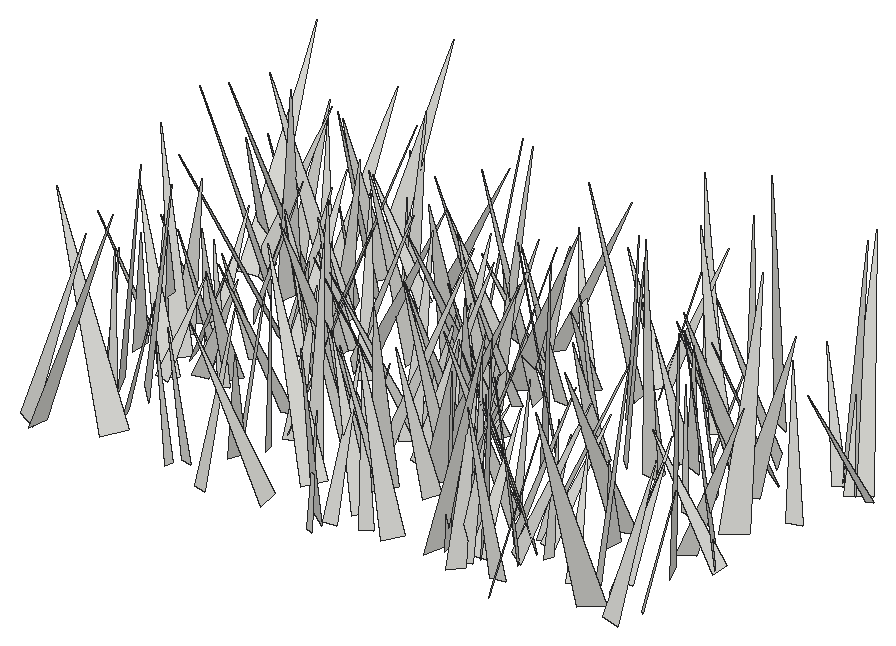
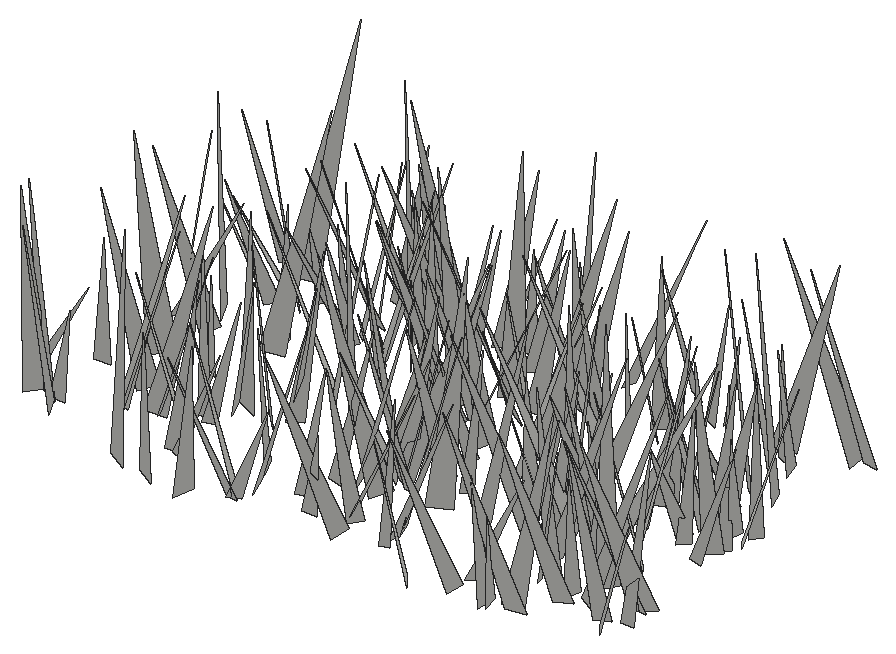
# SketchUp Ruby script. Lengths in inches.
U = 1.inch
M = Sketchup.active_model
def pt(a) = Geom::Point3d.new(a.map { |v| v * U })
def face(e, loops, mat)
  f = e.add_face(loops[0].map { |a| pt(a) })
  loops[1..].each { |l| e.add_face(l.map { |a| pt(a) }).erase! }
  f.material = f.back_material = mat if mat
  f
end
# faces: each face lists its corners as indices into pts; further lists are holes
def faces(e, pts, list, mat = nil) = list.each { |f| face(e, (f[0].is_a?(Array) ? f : [f]).map { |l| l.map { |i| pts[i] } }, mat) }
# xy, xz, yz: faces in a plane at the given z, y or x. An outline is a flat list of corners, or four numbers for a rectangle; further outlines are holes
def ring(l) = l.size == 4 ? [[l[0], l[1]], [l[2], l[1]], [l[2], l[3]], [l[0], l[3]]] : l.each_slice(2).to_a
def flat(e, list, mat, &to3) = list.each { |f| face(e, (f[0].is_a?(Array) ? f : [f]).map { |l| ring(l).map { |u, v| to3.(u, v) } }, mat) }
def xy(e, z, list, mat = nil) = flat(e, list, mat) { |x, y| [x, y, z] }
def xz(e, y, list, mat = nil) = flat(e, list, mat) { |x, z| [x, y, z] }
def yz(e, x, list, mat = nil) = flat(e, list, mat) { |y, z| [x, y, z] }
def lines(e, pts, list) = list.each { |a, b| e.add_line(pt(pts[a]), pt(pts[b])) }
# prism: a flat outline (further loops are holes) pulled along v
def prism(e, loops, v, mat = nil)
  f = face(e, loops, mat); d = Geom::Vector3d.new(v.map { |x| x * U })
  f.pushpull(f.normal.samedirection?(d) ? d.length : -d.length)
end
def box(e, o, s, mat = nil) = prism(e, [[o, [o[0] + s[0], o[1], o[2]], [o[0] + s[0], o[1] + s[1], o[2]], [o[0], o[1] + s[1], o[2]]]], [0, 0, s[2]], mat)
def at(x, y, z, deg = 0) = Geom::Transformation.translation(pt([x, y, z])) * Geom::Transformation.rotation(ORIGIN, Z_AXIS, deg.degrees)
def axes(o, x, y, z) = Geom::Transformation.new([*x, 0, *y, 0, *z, 0, *pt(o).to_a, 1])
def part(name) = M.definitions.add(name)
# library, detail: a bought-in or finely detailed component or shape, given as its bounding box
def library(name, o, s) = part(name).tap { |d| box(d.entities, o, s) }
def detail(e, o, s) = box(e.add_group.entities, o, s)
def put(e, d, t, mat = nil) = e.add_instance(d, t).tap { |i| i.material = mat if mat }
def group(e, t, mat = nil) = e.add_group.tap { |g| g.transformation = t; g.material = mat if mat }.entities
root = M.entities
c1 = part("fur_instance\#9")
p = [[0.8125,0,1.79],[0.67,-0.02,1.48],[0,-0.11,0],[0,0.11,0]]
faces(c1.entities,p,[[0,1,2,3]])
put(root,c1,axes([476.15,435.58,-21.66],[-2.86307,-5.78602,1.82095],[-5.78172,3.21211,1.11581],[1.83453,1.09334,6.35847]))
put(root,c1,axes([472.6,435.43,-21.66],[-6.27523,-0.24227,0.55286],[-0.1392,6.19931,1.13667],[0.58735,-1.11924,6.17618]))
put(root,c1,axes([495.21,437.4,-21.66],[3.52334,-7.25518,1.10129],[-7.15699,-3.66725,-1.26216],[-1.62106,0.42196,7.96608]))
put(root,c1,axes([476.77,434.08,-21.66],[1.67627,3.15128,1.04901],[3.10636,-1.90337,0.75402],[-1.17538,-0.53615,3.48882]))
put(root,c1,axes([455.6,434.11,-21.66],[2.77668,6.00015,1.42785],[6.14966,-2.57364,-1.14395],[0.47149,-1.76779,6.51177]))
put(root,c1,axes([456.45,434.12,-21.66],[7.58645,0.4489,1.20084],[0.2907,-7.62155,1.01257],[-1.24861,0.95304,7.53196]))
put(root,c1,axes([465.38,435.19,-21.66],[-3.65849,-0.26653,0.63033],[-0.40108,3.61269,-0.80033],[0.55452,0.85461,3.57982]))
put(root,c1,axes([468.625,434.03,-21.66],[1.97963,5.14738,0.61551],[5.06452,-2.06097,0.94673],[-1.10678,-0.22402,5.43306]))
put(root,c1,axes([466.03,435.98,-21.66],[-1.43157,-3.77915,1.63266],[-4.11341,1.2436,-0.72817],[-0.16553,1.78,3.97506]))
put(root,c1,axes([489.01,436.39,-21.66],[-0.52973,-5.32119,2.08202],[-5.65742,0.19488,-0.94137],[-0.8022,2.1395,5.26399]))
put(root,c1,axes([489.66,434.83,-21.66],[4.69636,2.95892,0.9191],[2.85112,-4.78039,0.82137],[-1.21287,0.21986,5.48965]))
put(root,c1,axes([481.15,436.42,-21.66],[-4.7653,3.97573,1.88545],[4.327,4.73874,0.94381],[0.79899,-1.95123,6.13381]))
put(root,c1,axes([460.6,436.08,-21.66],[-6.11884,4.72961,1.11538],[4.85918,5.97068,1.339],[0.0418,-1.7422,7.61686]))
put(root,c1,axes([467.91,438.375,-21.66],[4.2644,-2.86076,0.08373],[-2.8192,-4.22473,-0.76148],[-0.49304,-0.58632,5.07831]))
put(root,c1,axes([486.15,436.83,-21.66],[-1.6675,3.7386,1.84502],[3.94069,2.06209,-0.61692],[1.36097,-1.39013,4.04687]))
put(root,c1,axes([480.8125,436.93,-21.66],[-5.83458,-0.97839,0.23219],[-1.00024,5.78729,-0.74851],[0.10327,0.77686,5.8685]))
put(root,c1,axes([459.8,438.08,-21.66],[5.00049,1.26706,0.71261],[1.41038,-4.84715,-1.27832],[-0.35226,-1.4205,4.99762]))
put(root,c1,axes([483.9,436.83,-21.66],[7.6269,-0.50277,1.8471],[-0.68475,-7.80192,0.70374],[-1.78765,0.84341,7.61099]))
put(root,c1,axes([497.23,436.62,-21.66],[0.7475,5.23214,1.319],[5.34274,-0.53135,-0.92008],[0.75507,-1.41992,5.20456]))
put(root,c1,axes([486.23,435.9,-21.66],[-5.56085,2.56326,1.5764],[2.25423,5.74256,-1.38556],[1.99343,0.65656,5.96435]))
put(root,c1,axes([479.32,436.22,-21.66],[-0.14147,5.00237,0.6936],[4.87308,-0.04695,1.33257],[-1.32587,-0.70632,4.82369]))
put(root,c1,axes([477.17,435.48,-21.66],[0.66443,5.27954,0.01832],[5.19176,-0.65673,0.9642],[-0.95891,0.10252,5.2331]))
put(root,c1,axes([486.18,438.64,-21.66],[7.03768,2.72348,2.80411],[3.28727,-7.24831,-1.21043],[-2.11523,-2.20318,7.44856]))
put(root,c1,axes([477.89,437.65,-21.66],[-4.17135,3.80631,1.04328],[3.93898,4.10999,0.75433],[0.24669,-1.26356,5.59635]))
put(root,c1,axes([459.77,436.86,-21.66],[0.78619,5.10987,0.99795],[4.99569,-1.02461,1.31074],[-1.46621,-0.75112,5.00108]))
put(root,c1,axes([484.43,437.4375,-21.66],[-4.83197,-1.5354,1.95575],[-2.0901,4.8234,-1.3772],[1.34681,1.9768,4.87942]))
put(root,c1,axes([458.76,437.53,-21.66],[-4.7564,-0.43454,1.78324],[-0.95829,4.81251,-1.3833],[1.56539,1.62573,4.5715]))
put(root,c1,axes([488.3,440.76,-21.66],[-3.60567,-4.25836,0.82426],[-4.10665,3.69659,1.13335],[1.39586,-0.12438,5.46351]))
put(root,c1,axes([488.5625,438.86,-21.66],[3.89411,3.28531,3.07479],[3.51498,-4.75969,0.63397],[-2.80935,-1.40135,5.05524]))
put(root,c1,axes([477.09,440.71,-21.66],[5.45655,-4.97036,1.37233],[-4.9464,-5.60993,-0.6508],[-1.45634,0.43117,7.35221]))
put(root,c1,axes([483.26,438.07,-21.66],[6.3266,0.04535,0.7535],[-0.10627,-6.24313,1.26797],[-0.74735,1.27161,6.1984]))
put(root,c1,axes([473.5,438.63,-21.66],[-6.02819,4.2729,0.70004],[4.32885,5.97346,0.81585],[0.09372,-1.07093,7.34378]))
put(root,c1,axes([486.41,437.8,-21.66],[-2.91269,3.59929,0.76549],[3.33369,2.99435,-1.39463],[1.55801,0.3218,4.41516]))
put(root,c1,axes([485.46,438.91,-21.66],[-5.53054,0.45224,1.5037],[0.10523,5.59989,-1.29715],[1.5667,1.22031,5.39525]))
put(root,c1,axes([498.01,438.64,-21.66],[2.52886,2.74781,0.4271],[2.47453,-2.48701,1.34889],[-1.2687,0.62635,3.48225]))
put(root,c1,axes([488.21,439.12,-21.66],[2.55836,5.15566,0.46861],[5.11042,-2.43162,-1.14739],[0.82709,-0.92305,5.63999]))
put(root,c1,axes([492.64,438.85,-21.66],[-3.06168,2.49465,0.02952],[2.42804,2.99025,-0.87237],[0.57338,0.65813,3.85176]))
put(root,c1,axes([474.75,441.51,-21.66],[1.57492,-4.967,1.49516],[-5.0252,-1.8484,-0.84719],[-1.28605,1.13987,5.14138]))
put(root,c1,axes([457.36,440.77,-21.66],[6.90611,3.10223,2.59996],[3.46907,-7.18559,-0.64093],[-2.08547,-1.6797,7.5437]))
put(root,c1,axes([467.46,439.27,-21.66],[2.96652,3.66752,1.13191],[3.55325,-3.16507,0.94281],[-1.45132,-0.25254,4.62191]))
put(root,c1,axes([459.15,440.93,-21.66],[-4.14785,-5.45032,3.6874],[-5.74845,5.12259,1.10541],[3.20285,2.13555,6.75935]))
put(root,c1,axes([472.67,439.64,-21.66],[0.75585,6.87514,1.87347],[7.05211,-0.99202,0.79528],[-1.02238,-1.75986,6.87069]))
put(root,c1,axes([479.79,441.79,-21.66],[3.58153,-3.37168,2.12142],[-3.21603,-4.13077,-1.13573],[-2.3507,0.51427,4.78599]))
put(root,c1,axes([485.39,442.51,-21.66],[-6.52757,-2.25287,1.08541],[-2.07972,6.57544,1.14066],[1.38863,-0.74224,6.81054]))
put(root,c1,axes([468.82,440.18,-21.66],[3.80015,2.05854,2.10545],[1.83657,-4.34391,0.93228],[-2.30164,-0.0674,4.22014]))
put(root,c1,axes([495.16,439.14,-21.66],[3.38702,2.66566,0.2184],[2.51461,-3.29384,1.20529],[-0.91115,0.81867,4.13823]))
put(root,c1,axes([486.77,440.67,-21.66],[4.58071,3.98416,0.78034],[4.05613,-4.44078,-1.1369],[0.17387,-1.36793,5.96354]))
put(root,c1,axes([489.7,440.29,-21.66],[-4.04138,0.55951,1.25439],[0.25517,4.13619,-1.02282],[1.34961,0.89343,3.94964]))
put(root,c1,axes([493.64,440.01,-21.66],[4.42049,5.15695,1.86392],[5.12768,-4.73588,0.94203],[-1.94301,-0.76574,6.72662]))
put(root,c1,axes([478.75,443.38,-21.66],[3.49272,-6.19271,0.17705],[-6.11252,-3.41157,1.25629],[1.00898,0.76914,6.99789]))
put(root,c1,axes([484.67,443.94,-21.66],[-4.07639,-4.57708,0.71562],[-4.52519,4.13816,0.69067],[0.99219,0.06853,6.09012]))
put(root,c1,axes([494.95,440.8,-21.66],[-1.9043,4.31856,1.08738],[4.14528,2.15112,-1.28374],[1.62757,-0.42591,4.54184]))
put(root,c1,axes([488.14,441.73,-21.66],[-2.24113,2.46388,1.48853],[2.36542,2.65133,-0.82724],[1.6405,-0.45695,3.22631]))
put(root,c1,axes([491.23,445.45,-21.66],[2.31085,-7.14722,0.11909],[-7.10013,-2.30949,-0.83147],[-0.82765,-0.14321,7.46535]))
put(root,c1,axes([483.9375,441.61,-21.66],[2.37526,2.53476,1.46683],[2.25858,-2.78775,1.16004],[-1.86424,-0.14786,3.27432]))
put(root,c1,axes([481.07,441.62,-21.66],[1.22352,3.80068,0.33063],[3.61313,-1.04295,-1.38167],[1.22465,-0.72012,3.74608]))
put(root,c1,axes([473.85,441.8125,-21.66],[-6.46685,-0.99912,0.02995],[-0.985,6.33639,-1.3035],[-0.17003,1.29271,6.41243]))
put(root,c1,axes([469.26,441.91,-21.66],[-2.32023,4.26891,1.78267],[4.38145,2.66784,-0.68595],[1.48474,-1.20167,4.81004]))
put(root,c1,axes([491.71,443.85,-21.66],[3.65469,-1.69105,0.3912],[-1.57801,-3.61693,-0.89287],[-0.72291,-0.65395,3.92673]))
put(root,c1,axes([467.07,444.26,-21.66],[-0.62326,-5.57048,0.69706],[-5.46922,0.44429,-1.33972],[-1.26641,0.82277,5.44278]))
put(root,c1,axes([473.33,443.53,-21.66],[4.06757,1.21437,0.51699],[1.31683,-3.847,-1.32426],[-0.08902,-1.4188,4.03313]))
put(root,c1,axes([471.11,445.67,-21.66],[1.71301,-8.16044,0.92704],[-8.06805,-1.84913,-1.36891],[-1.53583,0.61199,8.22516]))
put(root,c1,axes([488.8,441.28,-21.66],[-0.26739,4.57604,0.32256],[4.40279,0.34673,-1.26925],[1.2883,-0.2352,4.40462]))
put(root,c1,axes([481.2,443.41,-21.66],[3.19088,3.17646,1.19509],[3.39239,-3.03309,-0.99593],[-0.09903,-1.55252,4.39087]))
put(root,c1,axes([462.09,445.4,-21.66],[3.35364,-3.87615,0.32814],[-3.76663,-3.34394,-1.00479],[-0.97195,-0.41544,5.02611]))
put(root,c1,axes([455.38,445.01,-21.66],[4.72712,-1.54603,0.79765],[-1.39638,-4.74943,-0.93014],[-1.03759,-0.65178,4.88576]))
put(root,c1,axes([478.71,444.61,-21.66],[-6.26748,-0.84521,1.62615],[-0.68504,6.45447,0.7145],[1.69984,-0.51518,6.28372]))
put(root,c1,axes([460.35,444.42,-21.66],[2.89103,-3.61881,0.35286],[-3.55779,-2.72252,1.22815],[0.74997,1.03461,4.46604]))
put(root,c1,axes([476.0625,445.86,-21.66],[-6.15592,-2.89241,0.11132],[-2.84807,6.09927,0.98037],[0.51666,-0.84058,6.73054]))
put(root,c1,axes([458.6875,442.88,-21.66],[-0.53064,3.51066,0.60828],[3.36851,0.69471,-1.0709],[1.16098,-0.41106,3.38519]))
put(root,c1,axes([496.49,443.375,-21.66],[6.19858,3.66698,3.16063],[3.75526,-6.8827,0.6206],[-3.05522,-1.01998,7.17523]))
put(root,c1,axes([468.73,445.13,-21.66],[-4.44854,-2.43941,1.67916],[-2.34276,4.75236,0.69742],[1.81157,0.15557,5.02532]))
put(root,c1,axes([458.98,443.23,-21.66],[-3.00084,5.06154,0.45444],[5.0055,2.85272,1.2797],[-0.87785,-1.03611,5.74339]))
put(root,c1,axes([468.4,442.87,-21.66],[6.55777,3.05775,0.67545],[3.00333,-6.58518,0.65252],[-0.88663,0.30968,7.20614]))
put(root,c1,axes([475.08,442.67,-21.66],[4.54632,6.46757,0.61256],[6.48609,-4.47646,-0.87508],[0.36794,-1.0028,7.85702]))
put(root,c1,axes([484.89,443.1875,-21.66],[-3.85021,0.78609,0.9669],[0.45373,3.80886,-1.28983],[1.16059,1.11875,3.71193]))
put(root,c1,axes([455.52,446.22,-21.66],[-3.97352,-3.33663,0.47318],[-3.25036,3.98768,0.8243],[0.89005,-0.33346,5.12275]))
put(root,c1,axes([498.41,445.36,-21.66],[-4.58076,1.47717,0.18742],[1.47131,4.39705,1.30451],[-0.22897,-1.29786,4.63288]))
put(root,c1,axes([462.17,444.32,-21.66],[-0.0394,4.36961,1.02441],[4.32756,-0.23455,1.1669],[-1.18959,-0.99797,4.2111]))
put(root,c1,axes([477.99,447.39,-21.66],[6.15158,-3.29467,0.71793],[-3.15743,-6.15236,-1.17953],[-1.18361,-0.7112,6.87789]))
put(root,c1,axes([459.72,446.73,-21.66],[-4.44345,-1.97155,1.25823],[-1.71315,4.58269,1.13072],[1.59225,-0.57131,4.72787]))
put(root,c1,axes([476.84,444.27,-21.66],[0.12132,5.40428,1.16344],[5.42728,0.10479,-1.05269],[1.05091,-1.16504,5.30215]))
put(root,c1,axes([458.5,446.12,-21.66],[4.5818,0.64032,0.1617],[0.65902,-4.5067,-0.82732],[-0.04299,-0.84188,4.55176]))
put(root,c1,axes([495.74,445.6,-21.66],[5.04993,-3.13211,0.88061],[-3.25342,-4.87587,1.31476],[-0.02926,1.58216,5.79512]))
put(root,c1,axes([455.91,447.3125,-21.66],[4.73789,-1.18845,0.72275],[-0.9672,-4.65874,-1.32025],[-0.99966,-1.12521,4.70287]))
put(root,c1,axes([497.93,445.66,-21.66],[-5.99226,-3.56649,1.99916],[-3.93709,5.99,-1.11487],[1.10264,2.00593,6.88361]))
put(root,c1,axes([477.34,445.52,-21.66],[6.84085,-1.05323,0.60817],[-1.14548,-6.7472,1.19982],[-0.40871,1.28156,6.81667]))
put(root,c1,axes([476.96,448.2,-21.66],[-0.56263,-5.96411,0.83016],[-5.9756,0.45013,-0.816],[-0.74291,0.89616,5.93475]))
put(root,c1,axes([485.75,446.46,-21.66],[5.05169,2.87341,0.23488],[2.86098,-4.93803,-1.1233],[0.35552,-1.09113,5.70213]))
put(root,c1,axes([485.0625,447.35,-21.66],[-5.96506,-5.04673,2.13711],[-5.35643,6.03696,-0.69462],[1.15994,1.92465,7.7826]))
put(root,c1,axes([456.51,445.57,-21.66],[-4.24883,1.88722,0.42776],[1.75815,4.19597,-1.04876],[0.80838,0.79335,4.52927]))
put(root,c1,axes([470.0625,449.52,-21.66],[-3.47678,-4.99975,0.07246],[-4.93171,3.44331,0.95532],[0.82523,-0.48669,6.01439]))
put(root,c1,axes([461.53,448.06,-21.66],[0.72019,-3.80208,0.86926],[-3.795,-0.88705,-0.73566],[-0.89965,0.69817,3.79912]))
put(root,c1,axes([458.27,448.2,-21.66],[3.6116,-2.54944,1.03868],[-2.46348,-3.75778,-0.65768],[-1.22872,0.0404,4.37159]))
put(root,c1,axes([458.01,445.59,-21.66],[-6.64184,2.29308,0.28161],[2.23011,6.58737,-1.04152],[0.60342,0.8944,6.94892]))
put(root,c1,axes([456.27,448.02,-21.66],[2.75053,-5.09352,1.52718],[-5.31748,-2.64324,0.76119],[-0.02665,1.70616,5.73847]))
put(root,c1,axes([482.7,448.56,-21.66],[6.58164,2.52237,2.667],[2.99732,-6.85363,-0.91486],[-2.11926,-1.85972,6.9888]))
put(root,c1,axes([474.63,446.14,-21.66],[-5.4201,3.31702,1.28358],[3.06796,5.54385,-1.37151],[1.7994,0.53923,6.20476]))
put(root,c1,axes([475.16,447.2,-21.66],[3.14685,5.37097,0.90824],[5.43729,-3.03382,-0.89816],[0.32882,-1.23429,6.15981]))
put(root,c1,axes([478.67,449.78,-21.66],[2.63547,-2.52355,0.88422],[-2.24578,-2.7628,-1.19134],[-1.45143,-0.30736,3.44888]))
put(root,c1,axes([465.74,449.32,-21.66],[0.59547,-6.22896,1.95156],[-6.50827,-0.41619,0.65745],[0.50087,1.99748,6.22272]))
put(root,c1,axes([456.4,449.44,-21.66],[-0.08918,-3.86635,0.81214],[-3.84672,-0.10019,-0.89937],[-0.90053,0.81086,3.76135]))
put(root,c1,axes([461.33,450.84,-21.66],[-3.69679,-5.87263,0.02895],[-5.78236,3.6339,-1.23044],[-1.02613,0.67962,6.82936]))
put(root,c1,axes([474,448.24,-21.66],[3.26385,-1.40609,1.47007],[-1.85279,-3.20219,1.05074],[-0.83985,1.59994,3.39496]))
put(root,c1,axes([458.75,447.47,-21.66],[-2.94733,3.27814,0.42411],[3.06608,2.92358,-1.29021],[1.23501,0.56503,4.21525]))
put(root,c1,axes([485.06,451.01,-21.66],[3.85472,-3.45884,0.89823],[-3.26491,-3.94586,-1.18314],[-1.45282,-0.30973,5.04209]))
put(root,c1,axes([464.62,450,-21.66],[2.18952,-4.24382,2.13551],[-4.35668,-2.73133,-0.96101],[-1.89466,1.3763,4.67766]))
put(root,c1,axes([476.07,452.03,-21.66],[-1.07248,-7.00957,0.36815],[-6.96342,1.01561,-0.94825],[-0.88342,0.50425,7.02746]))
put(root,c1,axes([471.96,451.31,-21.66],[3.81403,-1.87609,0.65313],[-1.66249,-3.78837,-1.17367],[-1.0874,-0.78844,4.08523]))
put(root,c1,axes([492.61,449.375,-21.66],[1.15906,3.62365,1.13013],[3.60388,-1.42153,0.86183],[-1.19166,-0.77453,3.7056]))
put(root,c1,axes([476.16,451.6,-21.66],[-4.22717,-2.44585,1.01456],[-2.28976,4.33627,0.91336],[1.32985,-0.3083,4.79759]))
put(root,c1,axes([465.16,451.66,-21.66],[3.88583,-1.17381,1.38743],[-0.79486,-4.04284,-1.19419],[-1.63432,-0.82466,3.87962]))
put(root,c1,axes([461.93,451.38,-21.66],[1.922,-3.18961,0.22781],[-3.1707,-1.86642,0.61867],[0.41494,0.51232,3.67219]))
put(root,c1,axes([496.3,449.35,-21.66],[5.95771,-4.00613,4.25574],[-5.13988,-6.48421,1.09155],[-2.78246,3.40011,7.09591]))
put(root,c1,axes([485.87,450.02,-21.66],[-5.27526,-0.92635,0.94955],[-1.13263,5.17215,-1.24665],[0.69057,1.40673,5.20887]))
put(root,c1,axes([465.16,452.16,-21.66],[3.57581,-3.48366,1.446],[-3.33217,-3.85124,-1.03819],[-1.76733,0.21279,4.88308]))
put(root,c1,axes([476.51,451.38,-21.66],[0.19192,-5.71021,2.24229],[-6.02696,-0.59408,-0.99702],[-1.14462,2.17066,5.62577]))
put(root,c1,axes([466.5,450.94,-21.66],[4.45392,4.12687,0.87812],[4.21021,-4.26347,-1.31776],[0.27618,-1.55927,5.92722]))
put(root,c1,axes([472.09,453.75,-21.66],[5.27875,-5.42072,0.96709],[-5.29735,-5.36505,-1.15714],[-1.50251,-0.12916,7.47733]))
put(root,c1,axes([468.1,450.17,-21.66],[-5.05186,2.37101,0.85511],[2.22237,5.09377,-0.9944],[1.18912,0.55319,5.49128]))
put(root,c1,axes([458.3,451.96,-21.66],[4.49917,3.28934,0.87918],[3.40387,-4.3112,-1.28935],[0.07989,-1.55853,5.42216]))
put(root,c1,axes([474.13,450.53,-21.66],[-1.65909,5.33475,1.21269],[5.33342,1.85943,-0.88312],[1.21852,-0.87506,5.51654]))
put(root,c1,axes([460.64,453.83,-21.66],[-0.56005,-4.94681,0.27227],[-4.82604,0.60667,1.09544],[1.12,0.14049,4.85639]))
put(root,c1,axes([461.46,451.71,-21.66],[0.44835,5.06558,1.88586],[5.29017,-0.02286,-1.19629],[1.10933,-1.93829,4.94267]))
put(root,c1,axes([463.05,449.94,-21.66],[-2.73527,5.15415,0.70761],[4.98067,2.82527,-1.3261],[1.50298,0.0175,5.68229]))
put(root,c1,axes([488.29,451.49,-21.66],[1.87849,6.8023,2.53671],[7.02619,-2.36292,1.13321],[-1.82724,-2.09291,6.96533]))
put(root,c1,axes([492.83,452.08,-21.66],[-3.64875,-2.02244,1.121],[-2.25149,3.58457,-0.86132],[0.52696,1.3118,4.08188]))
put(root,c1,axes([466.78,452.04,-21.66],[6.19791,-1.23637,0.25272],[-1.26158,-6.10069,1.0939],[-0.02993,1.12232,6.22464]))
put(root,c1,axes([476.96,453.25,-21.66],[-0.99125,-4.30354,0.98962],[-4.28593,0.69339,-1.27766],[-1.06332,1.21702,4.22737]))
put(root,c1,axes([488.79,451.95,-21.66],[-4.99068,-1.45127,1.21381],[-1.71677,4.91279,-1.18474],[0.79513,1.49823,5.06058]))
put(root,c1,axes([468.82,453.8,-21.66],[-6.42976,0.15301,2.02637],[0.5172,6.6259,1.14077],[1.96522,-1.24316,6.3296]))
put(root,c1,axes([489.66,453.73,-21.66],[-0.19463,-4.95849,1.24268],[-5.00803,0.4343,0.94858],[1.02496,1.18047,4.8708]))
put(root,c1,axes([457.09,455.1,-21.66],[-6.10704,-5.17922,1.29191],[-4.99805,6.23748,1.37932],[1.87424,-0.24245,7.88782]))
put(root,c1,axes([486.22,451.77,-21.66],[4.10758,4.73433,2.04961],[4.7509,-4.49256,0.85604],[-2.01089,-0.9434,6.20913]))
put(root,c1,axes([463.92,451.14,-21.66],[7.5502,3.19495,0.69372],[3.12341,-7.56468,0.84526],[-0.96605,0.51231,8.15468]))
put(root,c1,axes([494.09,455.81,-21.66],[-2.87377,-5.9267,0.11201],[-5.79461,2.83495,1.33509],[1.24935,-0.48389,6.44995]))
put(root,c1,axes([494.32,453.12,-21.66],[4.99795,-3.82327,1.26682],[-4.01963,-4.86241,1.18375],[-0.25457,1.71502,6.18026]))
put(root,c1,axes([492.01,455.34,-21.66],[1.78326,-6.33726,0.7797],[-6.26284,-1.89367,-1.06754],[-1.24322,0.44943,6.49625]))
put(root,c1,axes([498.36,452.41,-21.66],[-0.93822,4.8343,1.08723],[4.93478,0.81164,0.64956],[-0.44769,-1.18472,4.88147]))
put(root,c1,axes([474.6875,453.29,-21.66],[2.54446,5.11145,1.43196],[5.2695,-2.24073,-1.36501],[0.64019,-1.87187,5.54418]))
put(root,c1,axes([488.9,454.23,-21.66],[-2.91756,2.69263,1.56889],[3.08399,2.80363,0.92331],[0.448,-1.76443,3.86133]))
put(root,c1,axes([491.89,455.04,-21.66],[-4.72142,-2.258,0.83052],[-2.14472,4.77905,0.80066],[1.09019,-0.37724,5.17198]))
put(root,c1,axes([458.48,455.07,-21.66],[7.59105,-2.36712,2.02897],[-2.18853,-7.84946,-0.96967],[-2.22043,-0.35586,7.89221]))
put(root,c1,axes([475.72,454.625,-21.66],[6.5822,-3.48627,0.04021],[-3.46978,-6.5418,0.80411],[0.34104,0.72931,7.40492]))
put(root,c1,axes([475.91,452.6,-21.66],[3.67219,7.15908,2.03524],[7.27938,-3.92759,0.68132],[-1.55086,-1.48365,8.01705]))
put(root,c1,axes([476.24,452.45,-21.66],[4.4489,2.71988,0.66857],[2.4928,-4.41728,1.38241],[-1.27698,0.85286,5.02786]))
put(root,c1,axes([462.92,454.67,-21.66],[-8.06314,0.9505,0.88883],[1.02226,8.07835,0.63476],[0.80526,-0.7379,8.09412]))
put(root,c1,axes([478.76,455.12,-21.66],[-1.01611,-5.1437,1.43202],[-5.3112,0.8243,-0.80778],[-0.54728,1.55038,5.1805]))
put(root,c1,axes([477.5625,454.43,-21.66],[-7.02647,-2.17808,1.10616],[-2.29777,7.03636,-0.74079],[0.82938,1.04138,7.31892]))
put(root,c1,axes([461.85,455.89,-21.66],[0.25447,-5.59234,1.88155],[-5.79418,0.11887,1.13692],[1.11444,1.89496,5.48146]))
put(root,c1,axes([458.11,457.35,-21.66],[-3.1759,-6.57357,0.78945],[-6.61199,3.10387,-0.75436],[-0.34161,1.03711,7.26148]))
put(root,c1,axes([472.07,457.09,-21.66],[-5.80555,-2.80529,1.19859],[-2.69051,5.92298,0.83076],[1.43785,-0.24369,6.39405]))
put(root,c1,axes([493.05,457.66,-21.66],[-5.52274,-3.05851,1.02558],[-2.84433,5.57616,1.31266],[1.52186,-0.67738,6.17511]))
put(root,c1,axes([462.12,456.79,-21.66],[-3.33376,-1.76985,1.3611],[-1.54667,3.5947,0.88593],[1.61021,-0.21143,3.66899]))
put(root,c1,axes([489.58,455.76,-21.66],[4.36053,2.62617,0.62372],[2.69593,-4.29581,-0.7602],[-0.13318,-0.97427,5.03319]))
put(root,c1,axes([479.34,457.5625,-21.66],[2.09335,-3.21544,0.11512],[-3.16402,-2.08217,-0.6229],[-0.58423,-0.24481,3.78592]))
put(root,c1,axes([454.82,457.78,-21.66],[-0.80762,-5.18,0.70533],[-5.16495,0.90095,0.70267],[0.80822,0.5814,5.19528]))
put(root,c1,axes([500.17,457.18,-21.66],[-1.30366,-3.70433,0.26528],[-3.50778,1.13584,-1.37745],[-1.21983,0.69265,3.67753]))
put(root,c1,axes([475.5625,457.48,-21.66],[-4.15133,-1.53142,0.10873],[-1.49707,4.10736,0.69206],[0.34034,-0.61232,4.37033]))
put(root,c1,axes([455.28,456.05,-21.66],[2.30365,5.6713,0.71156],[5.64313,-2.13475,-1.25489],[0.90837,-1.12069,5.9913]))
put(root,c1,axes([471.88,458.2,-21.66],[-5.02334,-0.16728,0.55191],[-0.071,4.98153,0.86367],[0.57231,-0.85028,4.95137]))
put(root,c1,axes([482.89,456.28,-21.66],[-5.05417,-1.27819,2.14403],[-1.86511,5.15169,-1.32541],[1.65892,1.89778,5.04199]))
put(root,c1,axes([474.86,458.07,-21.66],[3.32524,-3.2763,0.88677],[-3.39381,-3.22791,0.80025],[-0.05063,1.1934,4.59902]))
put(root,c1,axes([471.7,459.36,-21.66],[-0.45629,-4.37673,0.42276],[-4.25435,0.54685,1.06962],[1.11127,0.29645,4.26847]))
put(root,c1,axes([487.93,458.4375,-21.66],[-0.66847,-3.61729,0.84651],[-3.58891,0.40659,-1.09666],[-0.95975,0.99906,3.51127]))
put(root,c1,axes([462.63,458.08,-21.66],[-3.17,-4.98135,1.74667],[-5.27871,2.99065,-1.05117],[-0.00204,2.03858,5.81015]))
put(root,c1,axes([459.54,457.01,-21.66],[-4.60941,2.24833,0.68921],[2.12734,4.63308,-0.88638],[1.00221,0.50623,5.05134]))
put(root,c1,axes([498.42,457.41,-21.66],[2.96295,7.07925,2.39249],[7.30087,-3.29107,0.69644],[-1.59283,-1.91622,7.64263]))
put(root,c1,axes([461.45,460.14,-21.66],[3.35042,-5.0359,1.55374],[-4.92978,-3.64566,-1.18576],[-1.86322,0.59037,5.93123]))
put(root,c1,axes([497.56,457.61,-21.66],[-1.2405,4.10694,0.41743],[4.03089,1.11105,1.04764],[-0.89058,-0.69186,4.16031]))
put(root,c1,axes([456.34,458.25,-21.66],[-0.43128,5.47544,2.09207],[5.72554,0.84273,-1.02531],[1.25517,-1.9628,5.39585]))
put(root,c1,axes([481.98,458.41,-21.66],[-6.45817,-1.9042,0.82118],[-2.02073,6.38203,-1.093],[0.4658,1.28531,6.64374]))
put(root,c1,axes([488.29,458.09,-21.66],[-2.02202,5.92033,1.45384],[6.05855,1.78151,1.17164],[-0.67672,-1.74024,6.14542]))
put(root,c1,axes([455.09,455.84,-21.66],[-3.2389,7.2108,0.31573],[7.08918,3.2432,-1.34571],[1.35602,0.26802,7.78942]))
put(root,c1,axes([465.25,459.27,-21.66],[-3.7614,2.09395,0.36046],[2.10674,3.58022,1.1859],[-0.27609,-1.20834,4.13841]))
put(root,c1,axes([499.21,457.36,-21.66],[-5.51425,5.90533,1.65371],[5.90522,5.71303,-0.71018],[1.6541,-0.70927,8.04832]))
put(root,c1,axes([455.72,459.22,-21.66],[-2.9488,-2.48385,0.84804],[-2.61567,2.88641,-0.64107],[0.2167,1.04076,3.80183]))
put(root,c1,axes([497.29,458.47,-21.66],[-5.34624,-2.21651,3.3319],[-3.00843,5.89263,-0.90721],[2.6389,2.22728,5.71596]))
put(root,c1,axes([482.57,459.68,-21.66],[4.81991,2.46867,0.79438],[2.57067,-4.76928,-0.77622],[-0.3421,-1.05666,5.35942]))
put(root,c1,axes([459.42,458,-21.66],[-0.94911,6.39885,1.08787],[6.32075,1.1611,-1.31509],[1.4754,-0.85797,6.33377]))
put(root,c1,axes([477.6,459.03,-21.66],[-1.23895,4.11427,0.01816],[3.97981,1.19363,1.09497],[-1.04341,-0.33255,4.15491]))
put(root,c1,axes([474.66,459.83,-21.66],[5.89255,-1.31891,0.46121],[-1.38894,-5.74659,1.31223],[-0.15186,1.38261,5.89404]))
put(root,c1,axes([482.22,460.29,-21.66],[-3.14834,2.92622,0.07201],[2.87738,3.07451,0.86494],[-0.53726,-0.68166,4.21031]))
put(root,c1,axes([465.36,460.71,-21.66],[5.25696,-1.00652,0.21452],[-1.02902,-5.15697,1.02054],[-0.01477,1.04274,5.25426]))
put(root,c1,axes([490.36,461.05,-21.66],[-3.60643,-6.53276,3.39182],[-7.2869,3.70246,-0.61691],[1.0404,3.28673,7.43658]))
put(root,c1,axes([482.3,460.4,-21.66],[1.86244,4.7215,0.55373],[4.68693,-1.72429,-1.06173],[0.79484,-0.89561,4.96326]))
put(root,c1,axes([462.66,460.78,-21.66],[-3.84179,0.25674,0.88435],[-0.00822,3.78425,-1.13434],[0.92083,1.10494,3.67947]))
put(root,c1,axes([462.88,460.97,-21.66],[-4.76791,1.69378,1.39092],[1.4281,4.92716,-1.10462],[1.66255,0.62512,4.93778]))
put(root,c1,axes([487.82,461.53,-21.66],[1.64216,5.46326,1.64146],[5.44457,-2.0108,1.24565],[-1.70244,-1.16093,5.56707]))
put(root,c1,axes([460.93,460.59,-21.66],[0.33819,7.69063,1.05021],[7.70297,-0.20312,-0.99305],[0.95553,-1.08446,7.63374]))
put(root,c1,axes([468.15,461.7,-21.66],[3.87453,3.49507,1.24049],[3.40824,-4.0629,0.80191],[-1.46226,-0.20898,5.15601]))
put(root,c1,axes([484.87,461.7,-21.66],[-6.05277,2.56522,0.71834],[2.46544,6.06973,-0.90131],[1.00895,0.55714,6.51184]))
